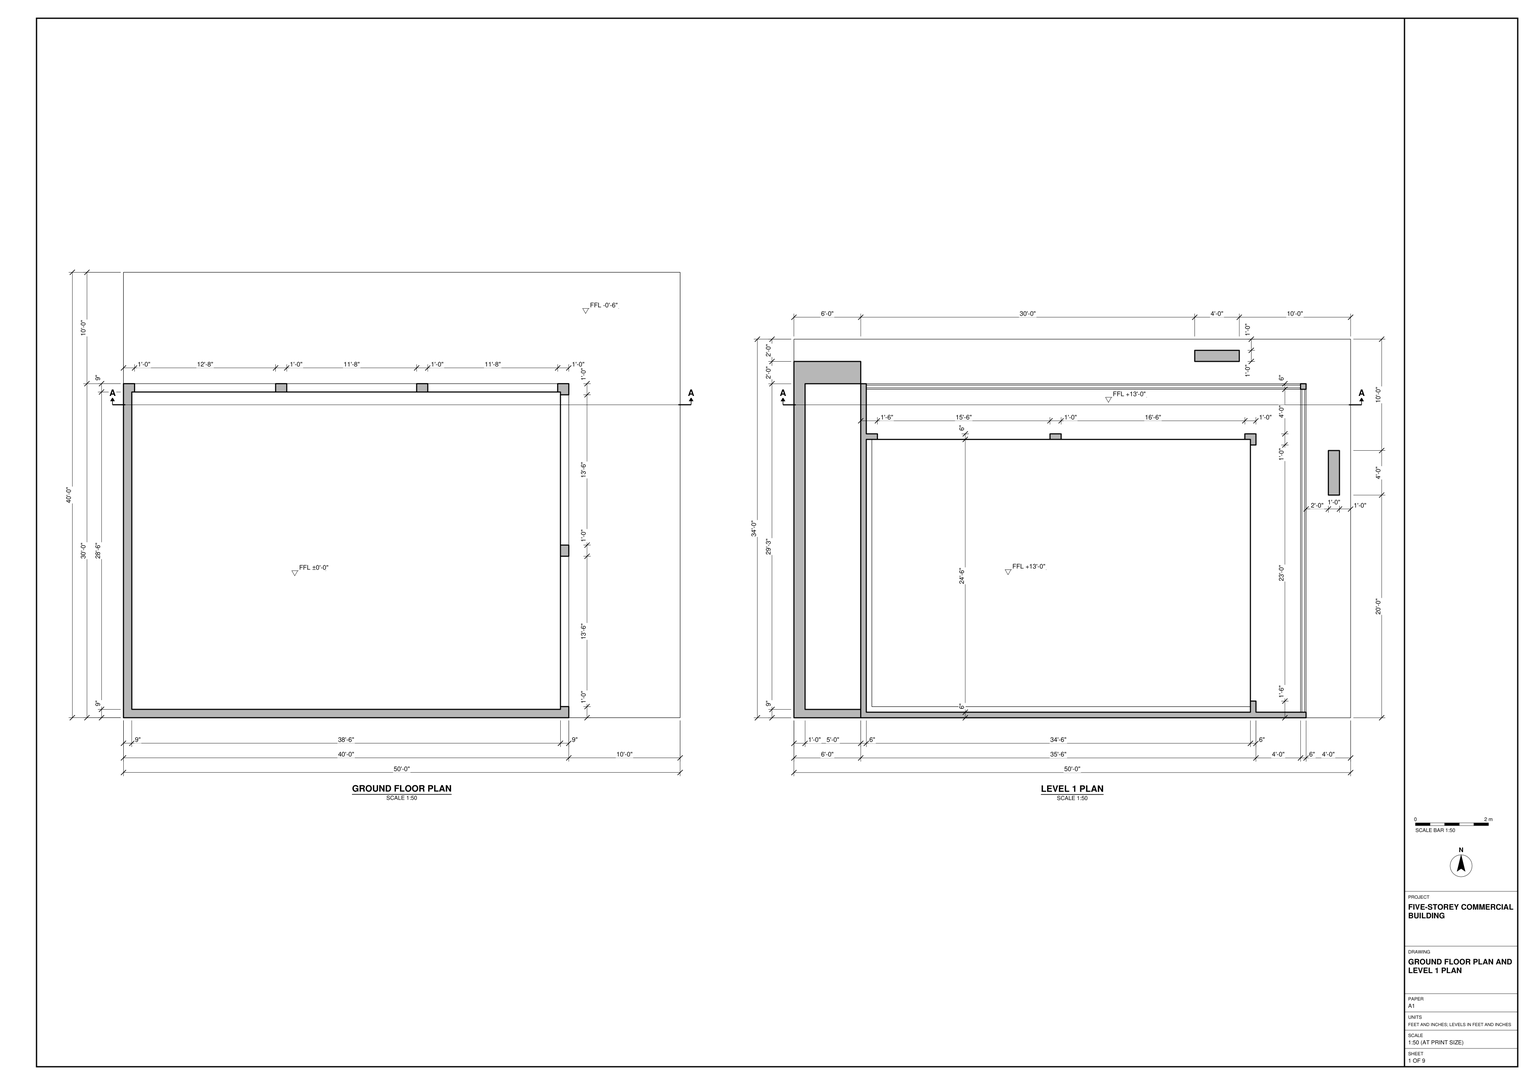
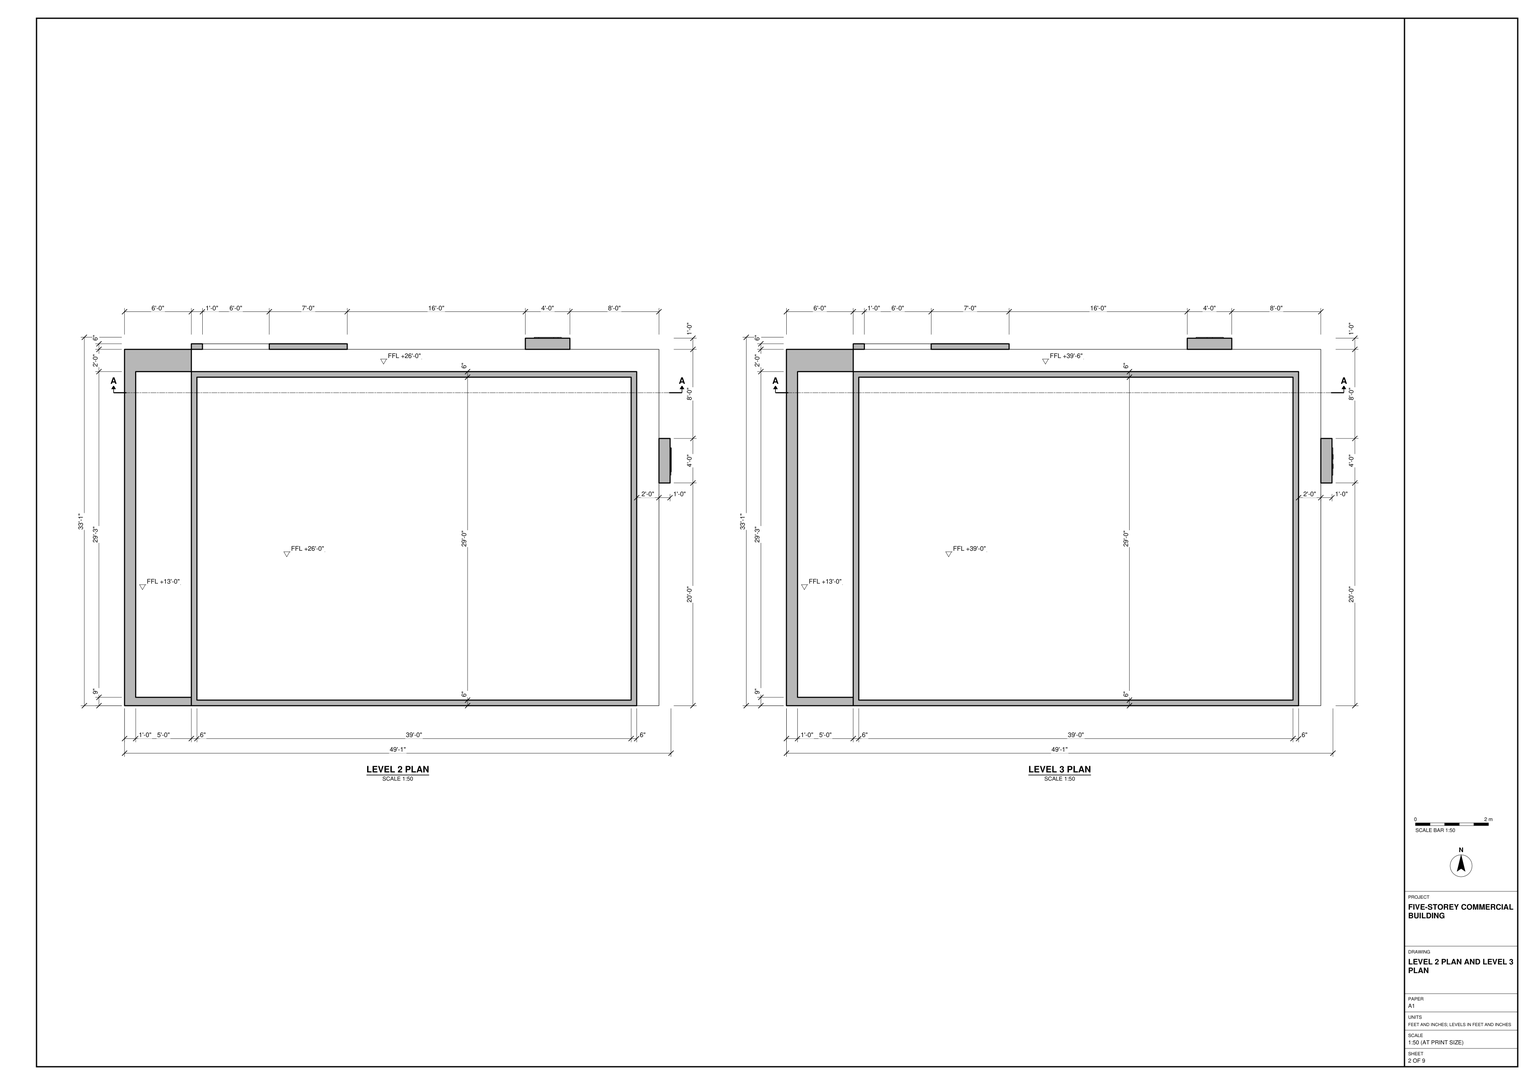
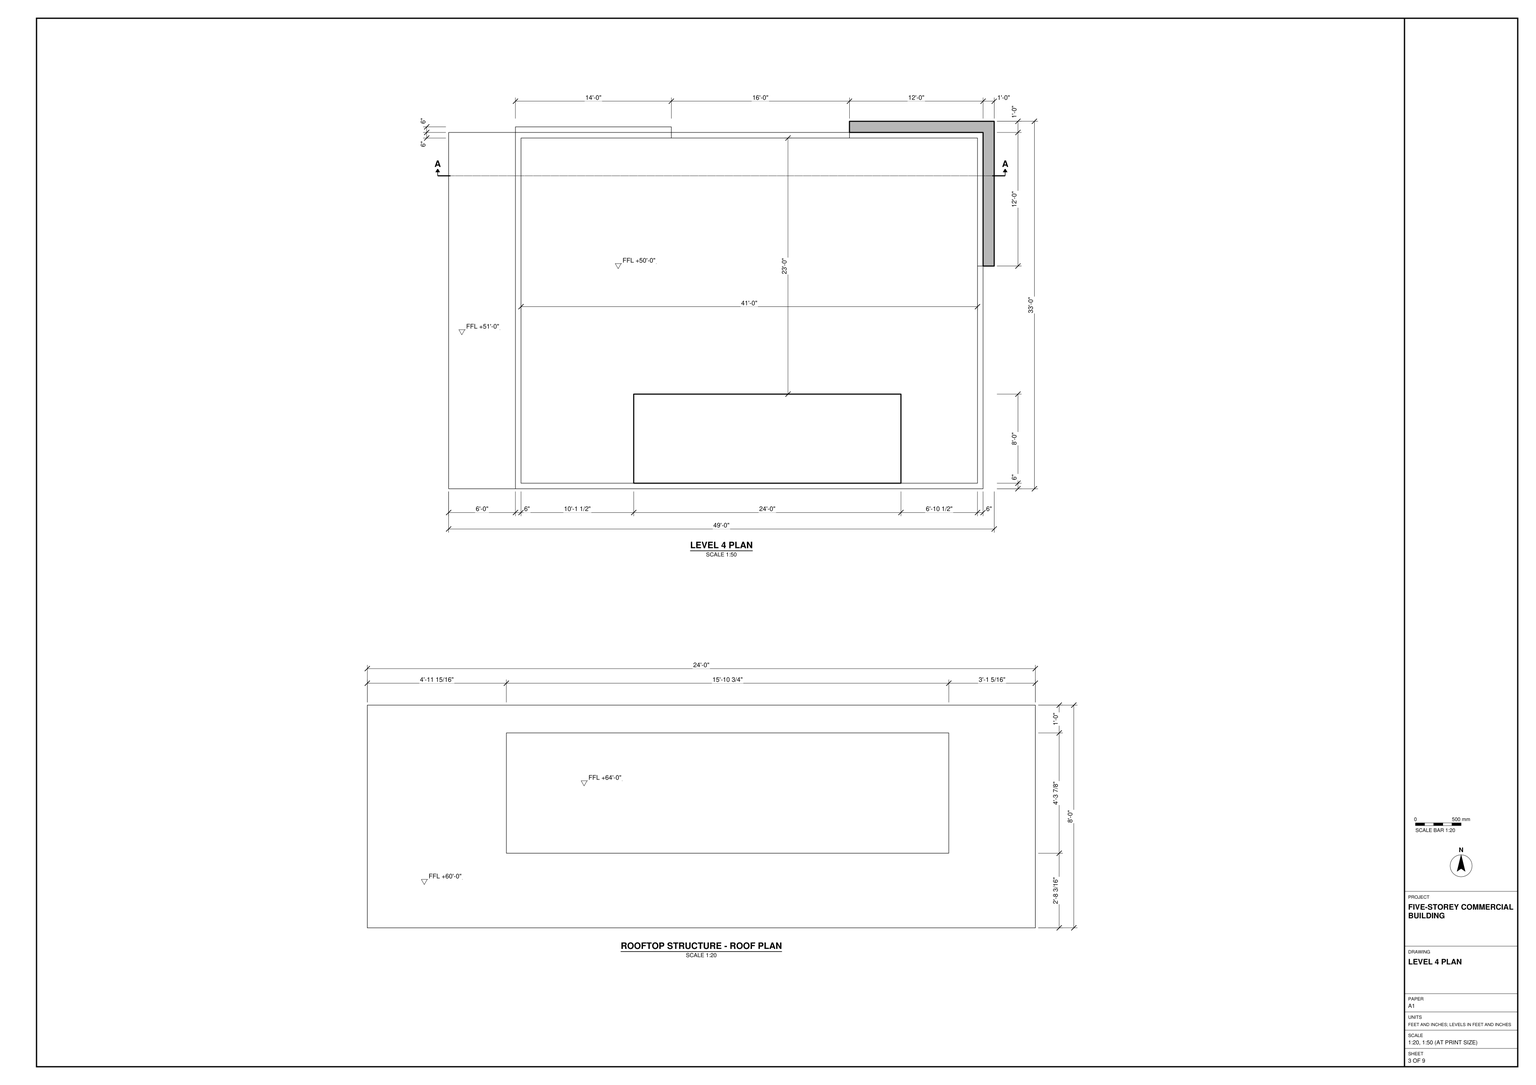
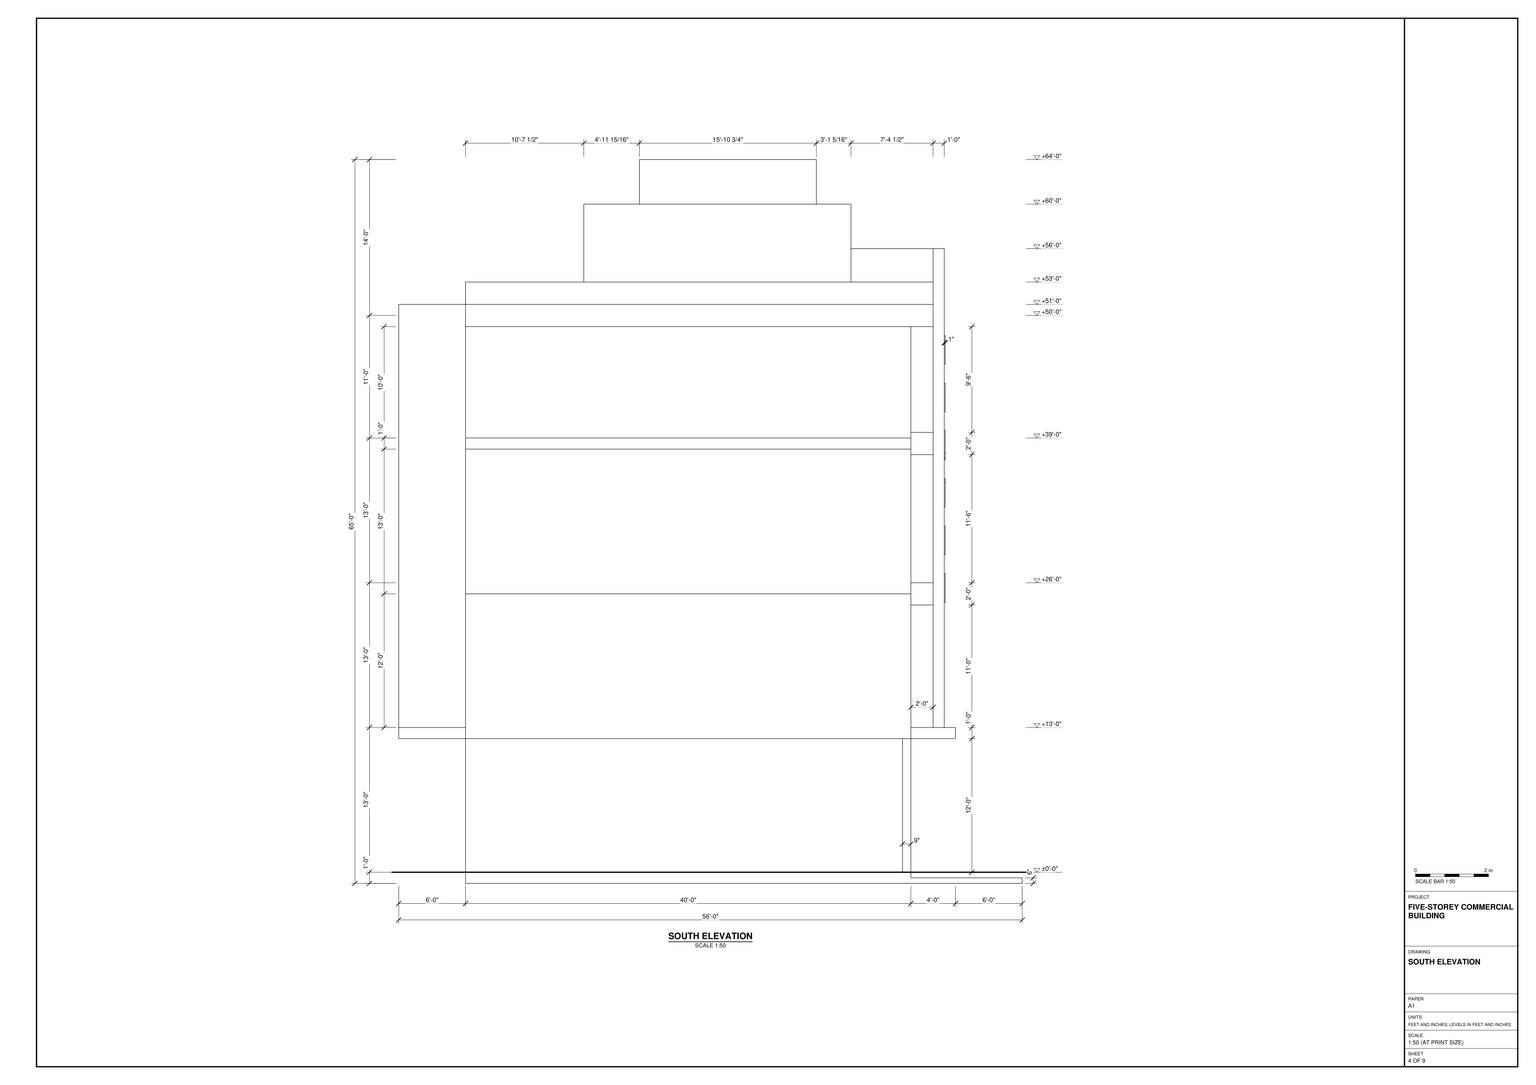
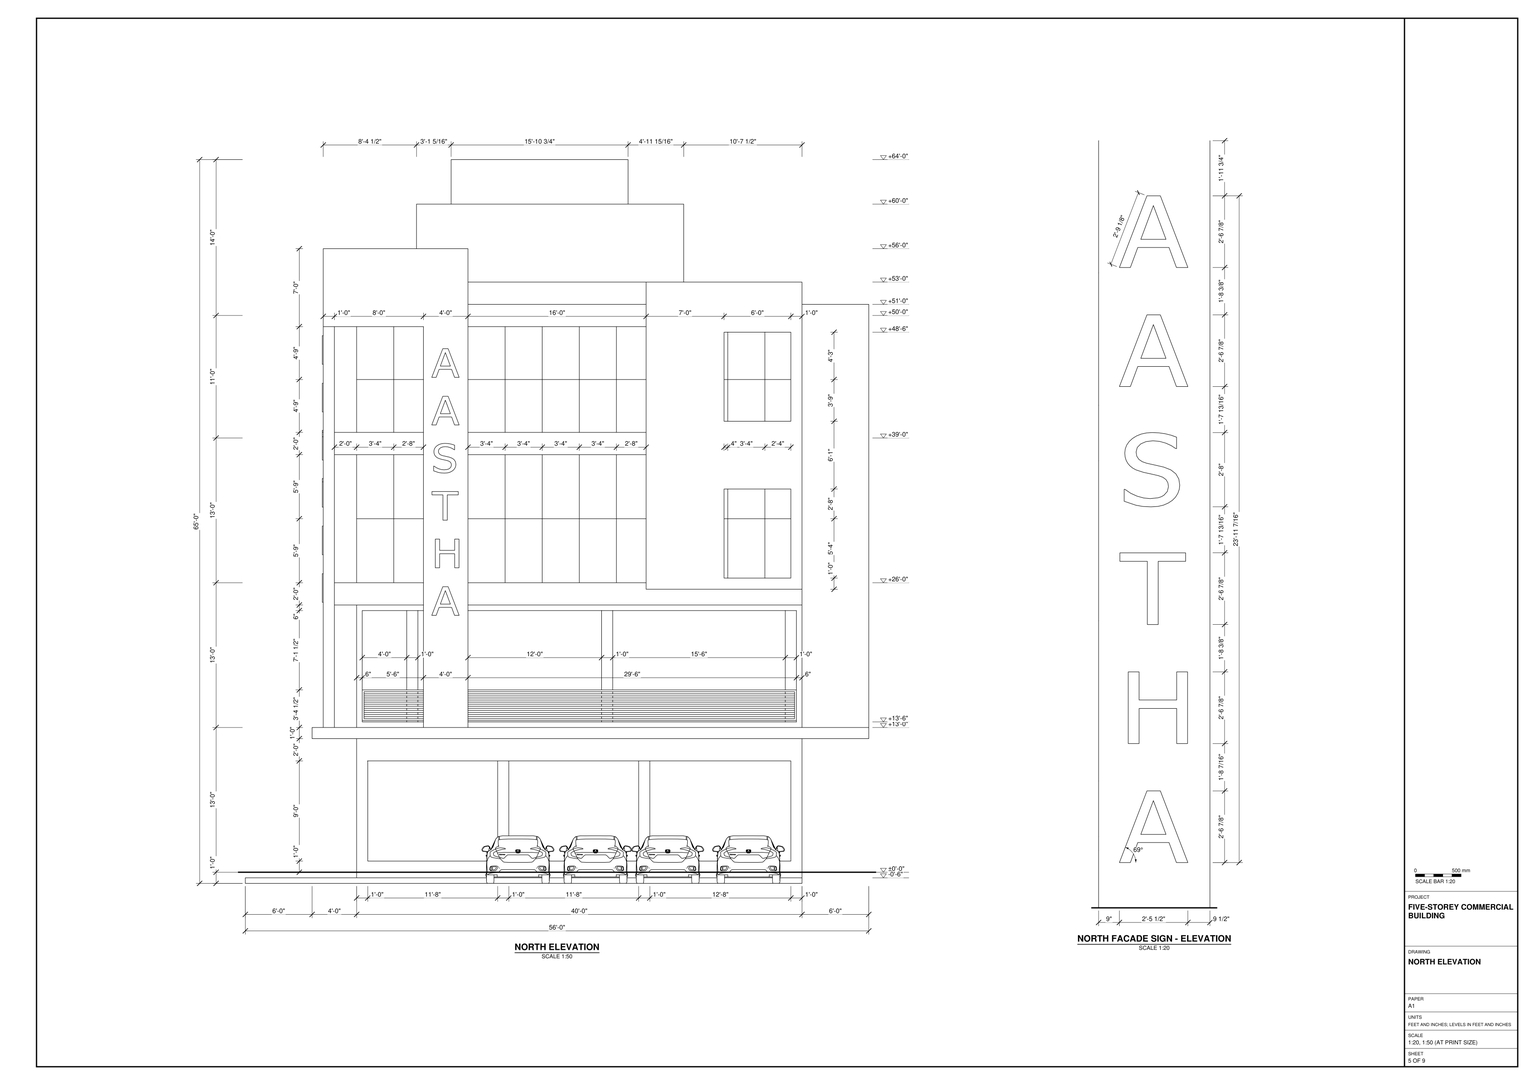
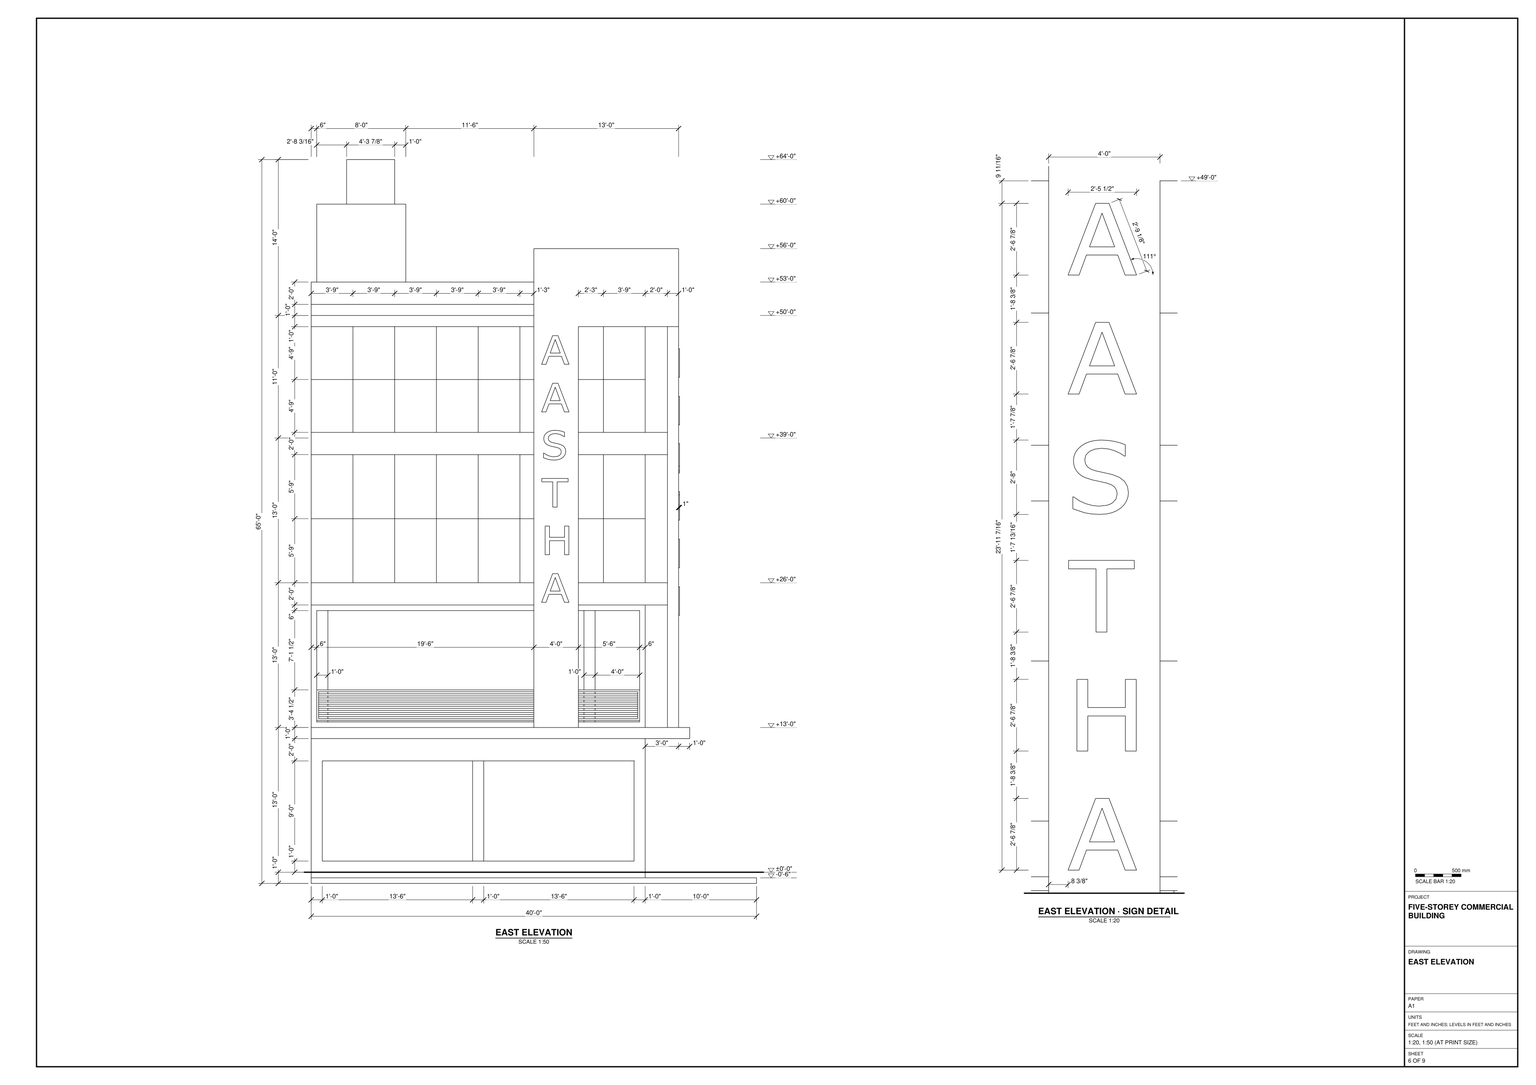
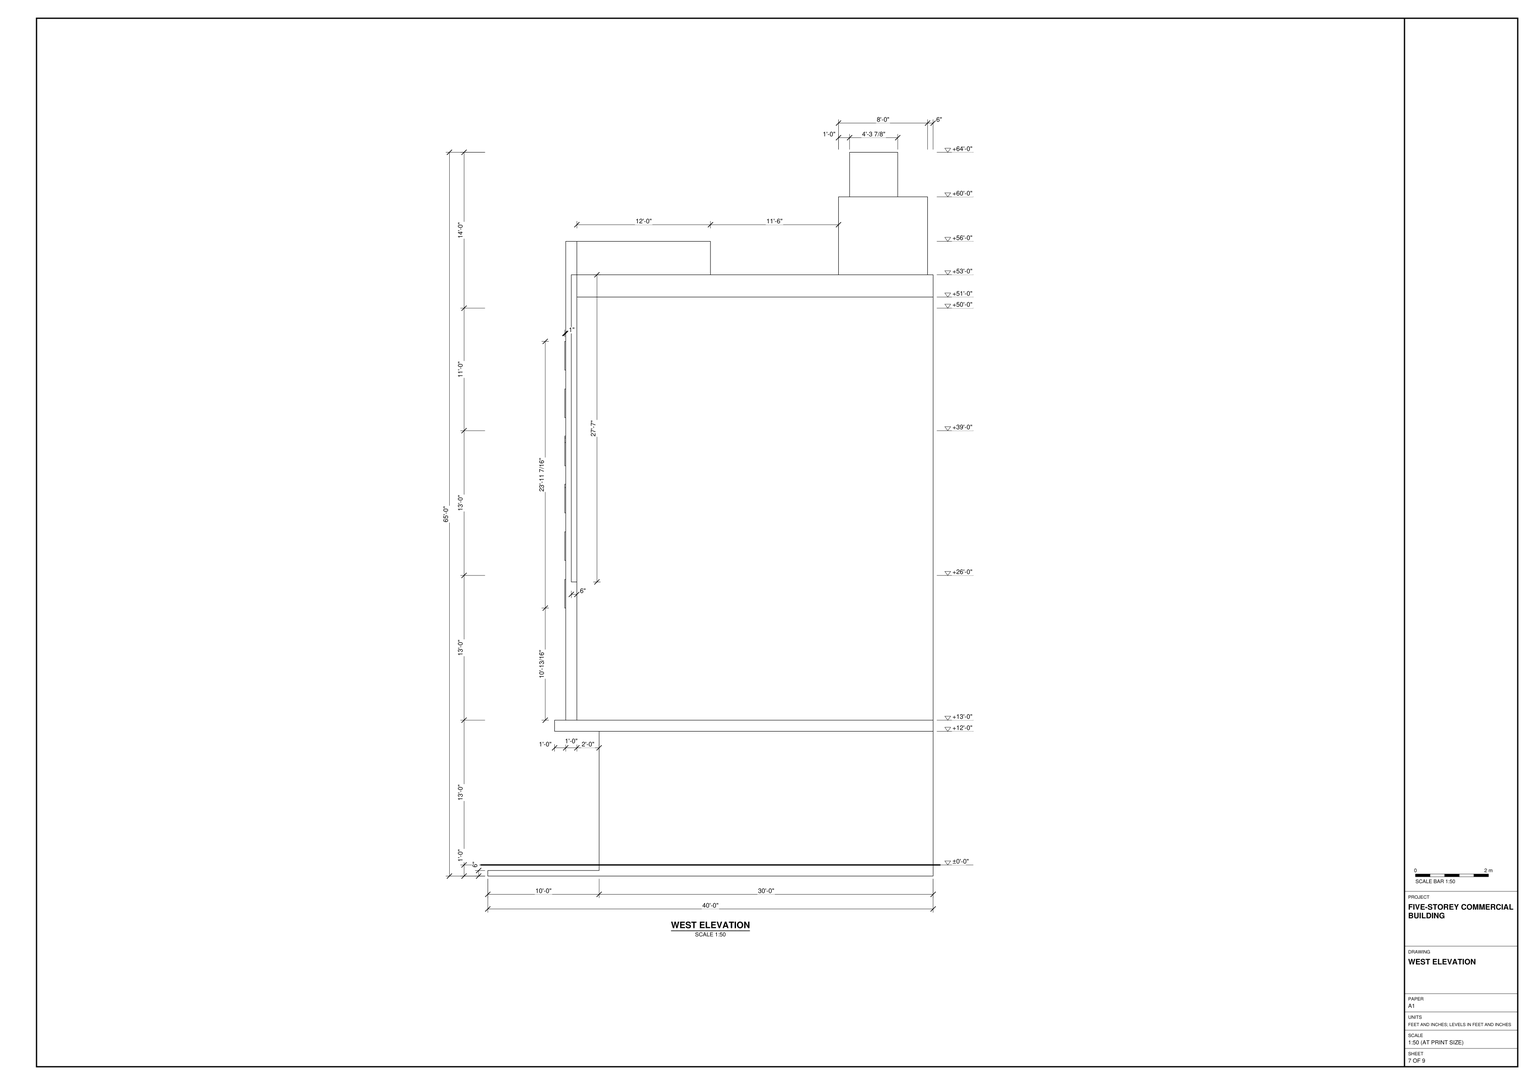
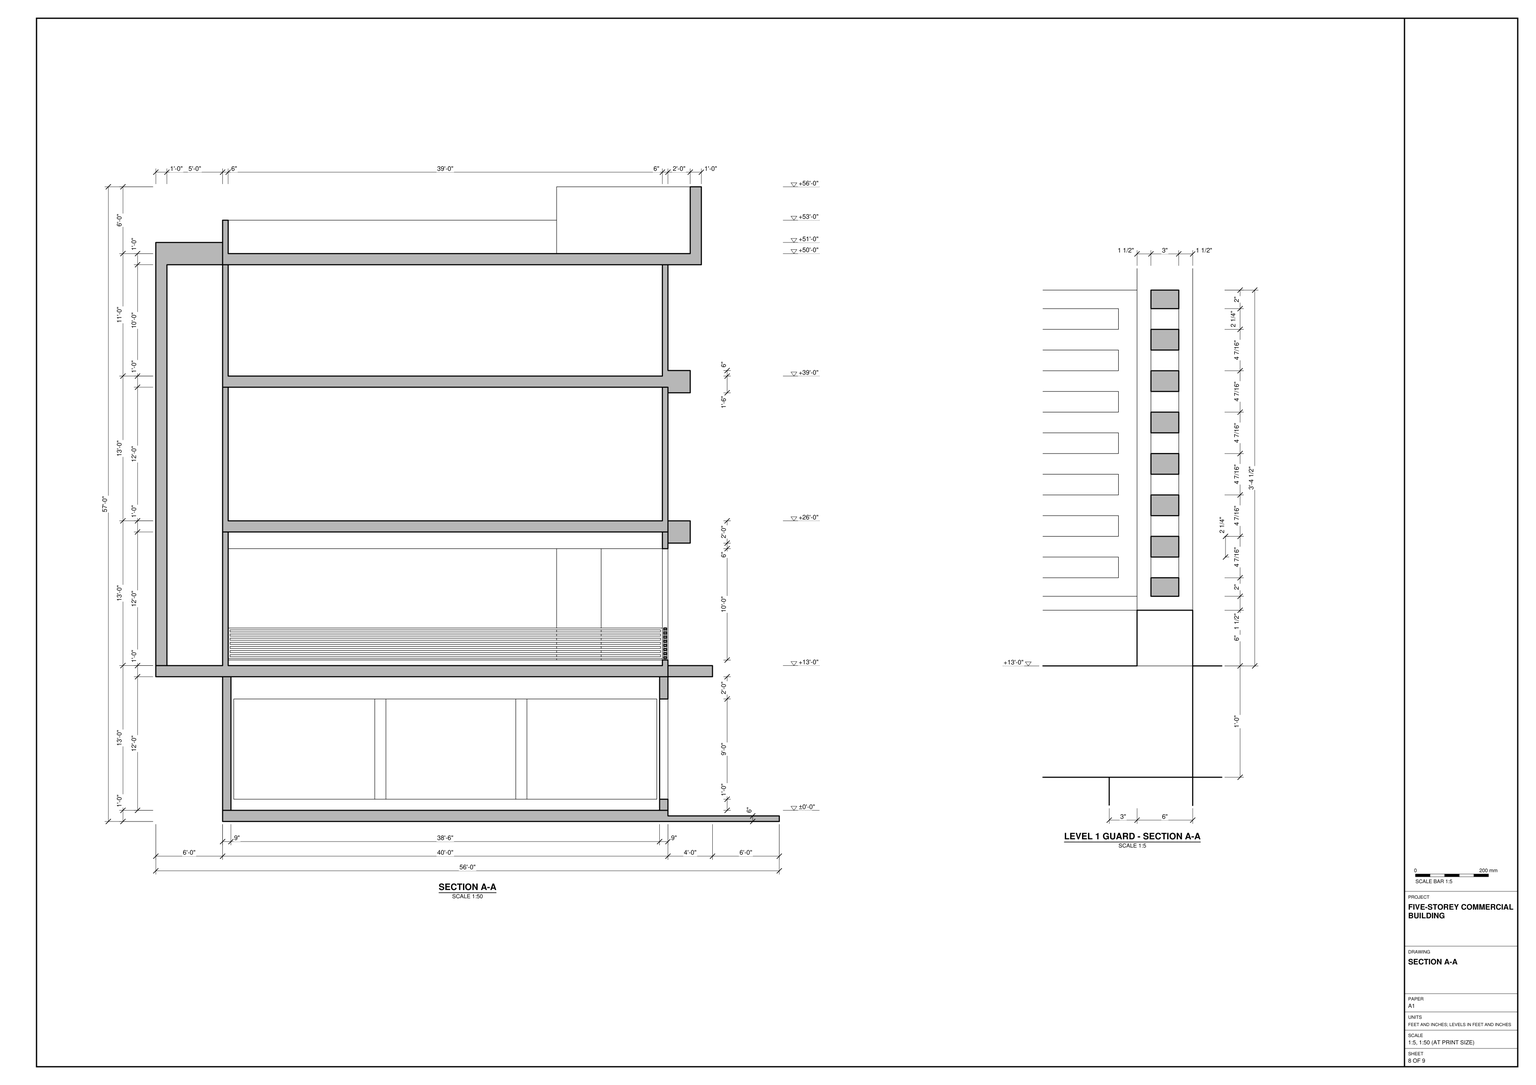
Build the commercial building in SketchUp from task_files/diagram_01.pdf. Work in feet and inches. The complete model must measure 56'-0" along X, 56'-2 9/16" along Y and 65'-0" along Z. Set the ground floor at ±0'-0" and Levels 1 through 4 at +13'-0", +26'-0", +39'-0" and +50'-0", respectively.

Place the rectangular ground-floor enclosure at the southwest corner of the base, leaving the exterior area shown to the north and east. Follow each floor plan for the slab edges, wall thicknesses, openings and perimeter supports. On Level 1, distinguish the enclosed floor area from the narrow bay to its west and the slab extending beyond it to the north and east. Use the matching enclosure outlines on Levels 2 and 3, keeping the west bay open to Level 1 below. On Level 4, model the roof perimeter and place the stepped rectangular rooftop structure along the south edge, with its smaller upper section inset as drawn.

Keep walls, slabs and roofs as separate groups or components, and do the same for each furniture or joinery piece shown. Use components for repeated parts. Decor and loose items may be any suitable library components. Save one SketchUp model as output_files/five_storey_commercial_building_with_stepped_rooftop.skp.

# SketchUp Ruby script. Lengths in inches.
U = 1.inch
M = Sketchup.active_model
def pt(a) = Geom::Point3d.new(a.map { |v| v * U })
def face(e, loops, mat)
  f = e.add_face(loops[0].map { |a| pt(a) })
  loops[1..].each { |l| e.add_face(l.map { |a| pt(a) }).erase! }
  f.material = f.back_material = mat if mat
  f
end
# faces: each face lists its corners as indices into pts; further lists are holes
def faces(e, pts, list, mat = nil) = list.each { |f| face(e, (f[0].is_a?(Array) ? f : [f]).map { |l| l.map { |i| pts[i] } }, mat) }
# xy, xz, yz: faces in a plane at the given z, y or x. An outline is a flat list of corners, or four numbers for a rectangle; further outlines are holes
def ring(l) = l.size == 4 ? [[l[0], l[1]], [l[2], l[1]], [l[2], l[3]], [l[0], l[3]]] : l.each_slice(2).to_a
def flat(e, list, mat, &to3) = list.each { |f| face(e, (f[0].is_a?(Array) ? f : [f]).map { |l| ring(l).map { |u, v| to3.(u, v) } }, mat) }
def xy(e, z, list, mat = nil) = flat(e, list, mat) { |x, y| [x, y, z] }
def xz(e, y, list, mat = nil) = flat(e, list, mat) { |x, z| [x, y, z] }
def yz(e, x, list, mat = nil) = flat(e, list, mat) { |y, z| [x, y, z] }
def lines(e, pts, list) = list.each { |a, b| e.add_line(pt(pts[a]), pt(pts[b])) }
# prism: a flat outline (further loops are holes) pulled along v
def prism(e, loops, v, mat = nil)
  f = face(e, loops, mat); d = Geom::Vector3d.new(v.map { |x| x * U })
  f.pushpull(f.normal.samedirection?(d) ? d.length : -d.length)
end
def box(e, o, s, mat = nil) = prism(e, [[o, [o[0] + s[0], o[1], o[2]], [o[0] + s[0], o[1] + s[1], o[2]], [o[0], o[1] + s[1], o[2]]]], [0, 0, s[2]], mat)
def at(x, y, z, deg = 0) = Geom::Transformation.translation(pt([x, y, z])) * Geom::Transformation.rotation(ORIGIN, Z_AXIS, deg.degrees)
def axes(o, x, y, z) = Geom::Transformation.new([*x, 0, *y, 0, *z, 0, *pt(o).to_a, 1])
def part(name) = M.definitions.add(name)
# library, detail: a bought-in or finely detailed component or shape, given as its bounding box
def library(name, o, s) = part(name).tap { |d| box(d.entities, o, s) }
def detail(e, o, s) = box(e.add_group.entities, o, s)
def put(e, d, t, mat = nil) = e.add_instance(d, t).tap { |i| i.material = mat if mat }
def group(e, t, mat = nil) = e.add_group.tap { |g| g.transformation = t; g.material = mat if mat }.entities
root = M.entities
M.materials.add("Glass_Basic_01").color = [0, 58, 107]
M.materials["Glass_Basic_01"].alpha = 0.58
M.materials.add("M05_Graphite_Haze").color = [114, 114, 114]
M.materials.add("M06_Steel_Smoke").color = [86, 86, 86]
c1 = library("2016+Honda+Civic+LX+Sedan",[0.01,0.03,0.02],[16.17,34.46,10.62])
c2 = library("A A S T H A",[-0.0625,0,0],[7.97,88.4375,1])
xz(root,300,[[90,168,276,300],[288,168,486,300]],"Glass_Basic_01")
xz(root,351,[[84,24,236,132],[248,24,388,132],[400,24,540,132]],"Glass_Basic_01")
yz(root,492,[[18,168,294,300]],"Glass_Basic_01")
yz(root,543,[[12,24,174,132],[186,24,348,132]],"Glass_Basic_01")
put(root,c1,axes([90.54,507.97,-0.09],[4.83,0,0],[0,4.83,0],[0,0,4.83]))
put(root,c1,axes([177.63,507.97,-0.09],[4.83,0,0],[0,4.83,0],[0,0,4.83]))
put(root,c1,axes([255.45,507.97,-0.09],[4.83,0,0],[0,4.83,0],[0,0,4.83]))
put(root,c1,axes([339.05,507.97,-0.09],[4.83,0,0],[0,4.83,0],[0,0,4.83]))
g1 = group(root,at(72,0,0))
xy(g1,0,[[0,0,600,480]])
xy(g1,6,[[480,0,600,0,600,480,0,480,0,360,480,360]])
xy(g1,156,[[-72,0,0,360],[0,0,480,360],[480,0,480,360,0,360,0,408,528,408,528,0],[-72,360,0,408]])
xy(g1,168,[[-72,0,-72,384,0,384,0,360,-60,360,-60,9,0,9,0,0],[[480,0,528,0,528,408,-72,408,-72,384,0,384,0,360,480,360],[504,240,516,288],[360,384,408,396]],[426,6,474,6,474,354,6,354,6,306,18,306,18,300,204,300,204,306,216,306,216,300,414,300,414,306,426,306,426,294,420,294,420,18,426,18],[6,6,420,6,420,12,12,12,12,300,6,300],[-60,9,0,360],
  [12,12,420,300]])
xy(g1,174,[[474,6,480,354],[6,354,474,360]])
xy(g1,175.5,[[475.5,6,478.5,354],[6,355.5,474,358.5]])
xy(g1,177.5,[[475.5,8,478.5,352],[8,355.5,472,358.5]])
xy(g1,179.73,[[475.5,8,478.5,352],[8,355.5,472,358.5]])
xy(g1,181.96,[[475.5,8,478.5,352],[8,355.5,472,358.5]])
xy(g1,184.19,[[475.5,8,478.5,352],[8,355.5,472,358.5]])
xy(g1,186.42,[[475.5,8,478.5,352],[8,355.5,472,358.5]])
xy(g1,188.65,[[475.5,8,478.5,352],[8,355.5,472,358.5]])
xy(g1,190.88,[[475.5,8,478.5,352],[8,355.5,472,358.5]])
xy(g1,193.12,[[475.5,8,478.5,352],[8,355.5,472,358.5]])
xy(g1,195.35,[[475.5,8,478.5,352],[8,355.5,472,358.5]])
xy(g1,197.58,[[475.5,8,478.5,352],[8,355.5,472,358.5]])
xy(g1,199.81,[[475.5,8,478.5,352],[8,355.5,472,358.5]])
xy(g1,202.04,[[475.5,8,478.5,352],[8,355.5,472,358.5]])
xy(g1,204.27,[[475.5,8,478.5,352],[8,355.5,472,358.5]])
xy(g1,206.5,[[475.5,8,478.5,352],[8,355.5,472,358.5]])
xy(g1,208.5,[[475.5,6,478.5,354],[6,355.5,474,358.5]])
xy(g1,294,[[474,6,480,354],[6,354,474,360]])
xy(g1,300,[[480,0,480,360,0,360,0,384,504,384,504,0]],"M05_Graphite_Haze")
xy(g1,300,[[420,18,426,294],[18,300,204,306],[204,300,216,306],[216,300,414,306]],"M06_Steel_Smoke")
xy(g1,312,[[0,0,480,6],[0,6,6,360],[420,6,426,6,426,306,6,306,6,300,420,300],[426,6,426,306,6,306,6,354,474,354,474,6],[6,6,420,300],
  [474,6,480,360],[6,354,474,360]])
xy(g1,316.99,[[0,384,168,390]])
xy(g1,324,[[6,6,474,354]])
xy(g1,324,[[480,0,504,0,504,384,0,384,0,360,480,360]],"M06_Steel_Smoke")
xy(g1,328.99,[[12,384,84,390]])
xy(g1,424.99,[[12,384,84,390]])
xy(g1,462,[[480,0,480,360,0,360,0,384,504,384,504,0]],"M05_Graphite_Haze")
xy(g1,468,[[0,0,6,360],[6,0,480,6],[6,6,474,354],[474,6,480,354],[6,354,480,360]])
xy(g1,480,[[6,6,474,354]])
xy(g1,486,[[480,0,504,0,504,384,0,384,0,360,480,360]],"M06_Steel_Smoke")
xy(g1,498,[[12,384,84,390]])
xy(g1,594,[[12,384,84,390]])
xy(g1,600,[[0,0,6,360],[6,0,474,6],[474,0,480,354],[6,6,474,354],[-60,9,0,360],
  [504,288,504,384,408,384,408,396,516,396,516,288],[6,354,480,360]])
xy(g1,600,[[480,0,480,360,0,360,0,384,504,384,504,0]],"M05_Graphite_Haze")
xy(g1,612,[[6,6,127.48,6,127.48,102,415.48,102,415.48,6,498,6,498,378,6,378],[498,240,504,240,504,384,360,384,360,378,498,378]])
xy(g1,624,[[-72,0,0,384]])
xy(g1,648,[[0,384,168,390]])
xy(g1,648,[[0,0,504,0,504,240,498,240,498,6,6,6,6,378,168,378,168,384,0,384],[168,378,360,384]],"M06_Steel_Smoke")
xy(g1,684,[[504,240,516,240,516,396,360,396,360,384,504,384]],"M06_Steel_Smoke")
xy(g1,732,[[[127.48,6,415.48,102],[187.44,38.17,378.17,90.03]]])
xy(g1,780,[[187.44,38.17,378.17,90.03]])
xz(g1,0,[[0,0,600,0,600,6,480,6,480,12,0,12],[-72,156,0,168],[0,156,480,312],[480,156,528,168],[-72,168,0,624],
  [0,312,480,468],[0,468,480,480],[0,480,480,600],[0,624,504,648]])
xz(g1,0,[[480,300,504,324],[480,462,504,486],[0,600,504,624]],"M06_Steel_Smoke")
xz(g1,6,[[6,168,420,312],[426,168,474,312],[[474,174,480,210],[475.5,175.5,478.5,208.5]],[474,210,480,294],[6,324,474,468],
  [6,480,474,600],[6,612,127.48,648],[415.48,612,498,648],[127.48,648,415.48,732]])
xz(g1,8,[[475.5,177.5,478.5,179.73],[475.5,181.96,478.5,184.19],[475.5,186.42,478.5,188.65],[475.5,190.88,478.5,193.12],[475.5,195.35,478.5,197.58],
  [475.5,199.81,478.5,202.04],[475.5,204.27,478.5,206.5]])
xz(g1,9,[[-60,168,0,600]])
xz(g1,18,[[420,168,426,300]],"M06_Steel_Smoke")
xz(g1,38.17,[[187.44,732,378.17,780]])
xz(g1,90.03,[[187.44,732,378.17,780]])
xz(g1,102,[[127.48,612,415.48,732]])
xz(g1,240,[[498,612,504,648]])
xz(g1,240,[[504,168,516,684]],"M06_Steel_Smoke")
xz(g1,288,[[504,168,516,600]])
xz(g1,294,[[420,168,426,300]],"M06_Steel_Smoke")
xz(g1,300,[[6,168,12,312]])
xz(g1,300,[[12,168,18,168,18,300,414,300,414,168,420,168,420,312,12,312],[204,168,216,300]],"M06_Steel_Smoke")
xz(g1,306,[[6,168,6,312,426,312,426,168,414,168,414,300,18,300,18,168],[204,168,216,300]],"M06_Steel_Smoke")
xz(g1,352,[[475.5,177.5,478.5,179.73],[475.5,181.96,478.5,184.19],[475.5,186.42,478.5,188.65],[475.5,190.88,478.5,193.12],[475.5,195.35,478.5,197.58],
  [475.5,199.81,478.5,202.04],[475.5,204.27,478.5,206.5]])
xz(g1,354,[[6,168,474,174],[[474,174,480,294],[475.5,175.5,478.5,208.5]],[6,294,474,312],[6,324,474,468],[6,480,474,600]])
xz(g1,355.5,[[[6,175.5,474,208.5],[8,181.96,472,184.19],[8,204.27,472,206.5],[8,199.81,472,202.04],[8,195.35,472,197.58],[8,190.88,472,193.12],[8,186.42,472,188.65],[8,177.5,472,179.73]]])
xz(g1,358.5,[[[6,175.5,474,208.5],[8,177.5,472,206.5]],[8,179.73,472,181.96],[8,184.19,472,186.42],[8,188.65,472,190.88],[8,193.12,472,195.35],
  [8,197.58,472,199.81],[8,202.04,472,204.27]])
xz(g1,360,[[0,6,480,12],[-60,168,0,600],[0,300,6,312],[6,300,474,312],[474,300,480,312],
  [0,312,480,324],[0,462,6,468],[6,462,480,468]])
xz(g1,360,[[0,324,40,393],[40,324,80,393],[80,324,120,393],[120,324,160,393],[160,324,200,393],
  [200,324,240,393],[240,324,280,393],[280,324,320,393],[320,324,360,393],[360,324,400,393],
  [400,324,440,393],[440,324,480,393],[0,393,40,462],[40,393,80,462],[80,393,120,462],
  [120,393,160,462],[160,393,200,462],[200,393,240,462],[240,393,280,462],[280,393,320,462],
  [320,393,360,462],[360,393,400,462],[400,393,440,462],[440,393,480,462],[0,486,40,543],
  [40,486,80,543],[80,486,120,543],[120,486,160,543],[160,486,200,543],[200,486,240,543],
  [240,486,280,543],[280,486,320,543],[320,486,360,543],[360,486,400,543],[400,486,440,543],
  [440,486,480,543],[0,543,40,600],[40,543,80,600],[80,543,120,600],[120,543,160,600],
  [160,543,200,600],[200,543,240,600],[240,543,280,600],[280,543,320,600],[320,543,360,600],
  [360,543,400,600],[400,543,440,600],[440,543,480,600]],"Glass_Basic_01")
xz(g1,360,[[[0,168,480,300],[6,174,474,294]]],"M06_Steel_Smoke")
xz(g1,378,[[6,612,360,648]])
xz(g1,384,[[360,168,408,300],[360,300,408,324],[[0,324,168,462],[12,328.99,84,424.99]],[360,324,408,462],[360,462,408,486],
  [[0,486,168,600],[12,498,84,594]],[360,486,408,600],[0,600,168,648],[360,600,504,612],[360,612,504,684],
  [168,624,360,648]])
xz(g1,384,[[-72,168,0,624],[0,300,0,316.99,168,316.99,168,324,360,324,360,300],[408,300,504,324],[0,316.99,168,324]],"M05_Graphite_Haze")
xz(g1,384,[[0,462,168,486],[168,462,360,486],[408,462,504,486],[168,600,360,624]],"M06_Steel_Smoke")
xz(g1,390,[[[0,316.99,168,648],[12,498,84,594],[12,328.99,84,424.99]]])
xz(g1,396,[[360,168,360,684,516,684,516,600,408,600,408,168]])
xz(g1,408,[[-72,156,528,168]])
xz(g1,480,[[0,0,600,6]])
yz(g1,-72,[[0,156,408,168],[0,168,384,624]])
yz(g1,-60,[[9,168,360,600]])
yz(g1,0,[[0,0,0,12,360,12,360,6,480,6,480,0],[0,168,9,312],[9,168,360,312],[0,312,9,468],[9,312,360,468],
  [384,316.99,390,648],[0,468,9,600],[9,468,360,600],[0,624,384,648]])
yz(g1,0,[[360,168,384,300],[360,324,384,462],[360,486,384,600]],"M05_Graphite_Haze")
yz(g1,0,[[360,300,384,324],[360,462,384,486],[0,600,360,624],[360,600,384,624]],"M06_Steel_Smoke")
yz(g1,6,[[6,168,300,312],[306,168,354,312],[[354,174,360,294],[355.5,175.5,358.5,208.5]],[6,324,354,468],[6,480,354,600],
  [6,612,378,648]])
yz(g1,8,[[355.5,177.5,358.5,179.73],[355.5,181.96,358.5,184.19],[355.5,186.42,358.5,188.65],[355.5,190.88,358.5,193.12],[355.5,195.35,358.5,197.58],
  [355.5,199.81,358.5,202.04],[355.5,204.27,358.5,206.5]])
yz(g1,12,[[384,328.99,390,424.99],[384,498,390,594]])
yz(g1,18,[[300,168,306,300]],"M06_Steel_Smoke")
yz(g1,84,[[384,328.99,390,424.99],[384,498,390,594]])
yz(g1,127.48,[[6,612,102,732]])
yz(g1,168,[[384,316.99,390,648]])
yz(g1,187.44,[[38.17,732,90.03,780]])
yz(g1,204,[[300,168,306,300]],"M06_Steel_Smoke")
yz(g1,216,[[300,168,306,300]],"M06_Steel_Smoke")
yz(g1,360,[[378,612,384,648]])
yz(g1,360,[[384,168,396,684]],"M06_Steel_Smoke")
yz(g1,378.17,[[38.17,732,90.03,780]])
yz(g1,408,[[384,168,396,600]])
yz(g1,414,[[300,168,306,300]],"M06_Steel_Smoke")
yz(g1,415.48,[[6,612,102,732]])
yz(g1,420,[[6,168,12,312]])
yz(g1,420,[[12,168,12,312,300,312,300,168,294,168,294,300,18,300,18,168]],"M06_Steel_Smoke")
yz(g1,426,[[6,168,18,168,18,300,294,300,294,168,306,168,306,312,6,312]],"M06_Steel_Smoke")
yz(g1,472,[[355.5,177.5,358.5,179.73],[355.5,181.96,358.5,184.19],[355.5,186.42,358.5,188.65],[355.5,190.88,358.5,193.12],[355.5,195.35,358.5,197.58],
  [355.5,199.81,358.5,202.04],[355.5,204.27,358.5,206.5]])
yz(g1,474,[[6,168,354,174],[[354,174,360,210],[355.5,175.5,358.5,208.5]],[354,210,360,294],[6,294,354,312],[6,324,354,468],
  [6,480,354,600]])
yz(g1,475.5,[[[6,175.5,354,208.5],[8,181.96,352,184.19],[8,204.27,352,206.5],[8,199.81,352,202.04],[8,195.35,352,197.58],[8,190.88,352,193.12],[8,186.42,352,188.65],[8,177.5,352,179.73]]])
yz(g1,478.5,[[[6,175.5,354,208.5],[8,177.5,352,206.5]],[8,179.73,352,181.96],[8,184.19,352,186.42],[8,188.65,352,190.88],[8,193.12,352,195.35],
  [8,197.58,352,199.81],[8,202.04,352,204.27]])
yz(g1,480,[[0,6,360,12],[0,156,360,168],[0,300,6,312],[6,300,360,312],[0,312,360,324],
  [0,462,6,468],[6,462,354,468],[354,462,360,468]])
yz(g1,480,[[0,324,45,393],[45,324,90,393],[90,324,135,393],[135,324,180,393],[180,324,225,393],
  [225,324,270,393],[270,324,315,393],[315,324,360,393],[0,393,45,462],[45,393,90,462],
  [90,393,135,462],[135,393,180,462],[180,393,225,462],[225,393,270,462],[270,393,315,462],
  [315,393,360,462],[0,486,45,543],[45,486,90,543],[90,486,135,543],[135,486,180,543],
  [180,486,225,543],[225,486,270,543],[270,486,315,543],[315,486,360,543],[0,543,45,600],
  [45,543,90,600],[90,543,135,600],[135,543,180,600],[180,543,225,600],[225,543,270,600],
  [270,543,315,600],[315,543,360,600]],"Glass_Basic_01")
yz(g1,480,[[[0,168,360,300],[6,174,354,294]]],"M06_Steel_Smoke")
yz(g1,498,[[6,612,240,648]])
yz(g1,504,[[240,168,288,300],[240,300,288,324],[240,324,288,462],[240,462,288,486],[240,486,288,600],
  [240,612,384,684],[0,624,240,648]])
yz(g1,504,[[0,300,240,324],[288,300,384,324],[0,462,240,486],[288,462,384,486],[0,600,240,612],
  [0,612,240,624]],"M06_Steel_Smoke")
yz(g1,516,[[240,168,288,168,288,600,396,600,396,684,240,684]])
yz(g1,528,[[0,156,408,168]])
yz(g1,600,[[0,0,480,6]])
p = [[480,360,468],[480,360,480]]
lines(g1,p,[[0,1]])
put(g1,c2,axes([516,248.6,302.875],[0,3.7052,0],[0,0,3.25],[1,0,0]),"M06_Steel_Smoke")
put(g1,c2,axes([398.8,396,288.8],[-3.7052,0,0],[0,0,3.25],[0,1,0]),"M06_Steel_Smoke")
g2 = group(g1,at(0,0,12))
xy(g2,0,[[[0,0,480,360],[9,9,471,351]],[9,9,471,351]])
xy(g2,12,[[471,174,480,186],[164,351,176,360],[316,351,328,360]])
xy(g2,12,[[471,12,480,174],[471,186,480,348],[12,351,164,360],[176,351,316,360],[328,351,468,360]],"M06_Steel_Smoke")
xy(g2,120,[[471,174,480,186],[164,351,176,360],[316,351,328,360]])
xy(g2,120,[[471,12,480,174],[471,186,480,348],[12,351,164,360],[176,351,316,360],[328,351,468,360]],"M06_Steel_Smoke")
xy(g2,144,[[[0,0,480,360],[9,9,471,351]]])
xz(g2,0,[[0,0,471,144],[471,0,480,144]])
xz(g2,9,[[9,0,471,144]])
xz(g2,12,[[471,12,480,120]],"M06_Steel_Smoke")
xz(g2,174,[[471,12,480,120]])
xz(g2,186,[[471,12,480,120]],"M06_Steel_Smoke")
xz(g2,348,[[471,12,480,120]])
xz(g2,351,[[[9,0,471,144],[12,12,468,120]],[164,12,176,120],[316,12,328,120]])
xz(g2,360,[[[0,0,480,144],[12,12,468,120]],[164,12,176,120],[316,12,328,120]],"M06_Steel_Smoke")
yz(g2,0,[[0,0,360,144]])
yz(g2,9,[[9,0,351,144]])
yz(g2,12,[[351,12,360,120]],"M06_Steel_Smoke")
yz(g2,164,[[351,12,360,120]])
yz(g2,176,[[351,12,360,120]],"M06_Steel_Smoke")
yz(g2,316,[[351,12,360,120]])
yz(g2,328,[[351,12,360,120]],"M06_Steel_Smoke")
yz(g2,468,[[351,12,360,120]])
yz(g2,471,[[[9,0,351,144],[12,12,348,120]],[174,12,186,120]])
yz(g2,480,[[[0,0,360,144],[12,12,348,120]],[174,12,186,120]],"M06_Steel_Smoke")
p = [[480,348,120],[468,360,120]]
lines(g2,p,[[0,1]])
